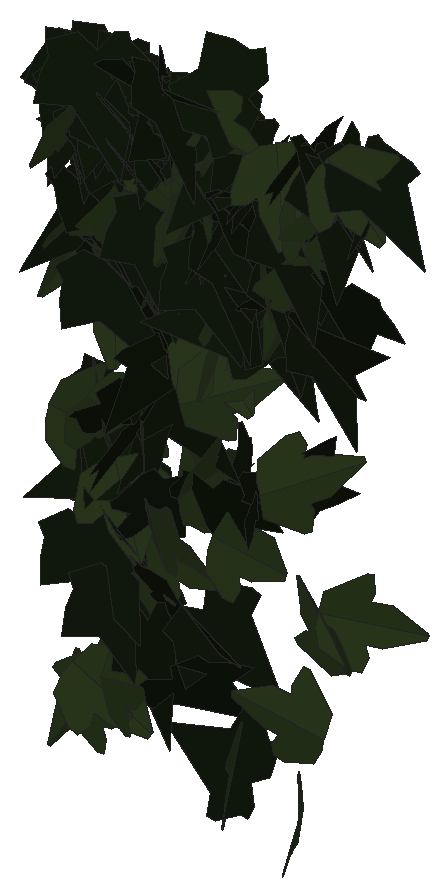
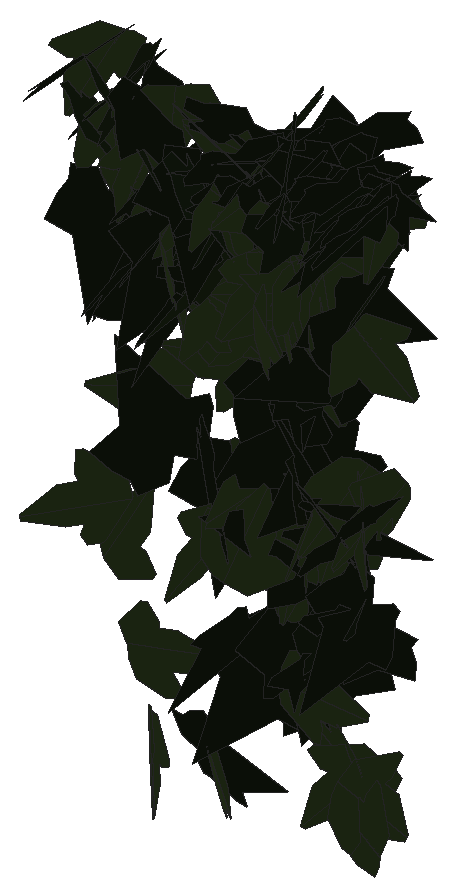
# SketchUp Ruby script. Lengths in inches.
U = 1.inch
M = Sketchup.active_model
def pt(a) = Geom::Point3d.new(a.map { |v| v * U })
def face(e, loops, mat)
  f = e.add_face(loops[0].map { |a| pt(a) })
  loops[1..].each { |l| e.add_face(l.map { |a| pt(a) }).erase! }
  f.material = f.back_material = mat if mat
  f
end
# faces: each face lists its corners as indices into pts; further lists are holes
def faces(e, pts, list, mat = nil) = list.each { |f| face(e, (f[0].is_a?(Array) ? f : [f]).map { |l| l.map { |i| pts[i] } }, mat) }
# xy, xz, yz: faces in a plane at the given z, y or x. An outline is a flat list of corners, or four numbers for a rectangle; further outlines are holes
def ring(l) = l.size == 4 ? [[l[0], l[1]], [l[2], l[1]], [l[2], l[3]], [l[0], l[3]]] : l.each_slice(2).to_a
def flat(e, list, mat, &to3) = list.each { |f| face(e, (f[0].is_a?(Array) ? f : [f]).map { |l| ring(l).map { |u, v| to3.(u, v) } }, mat) }
def xy(e, z, list, mat = nil) = flat(e, list, mat) { |x, y| [x, y, z] }
def xz(e, y, list, mat = nil) = flat(e, list, mat) { |x, z| [x, y, z] }
def yz(e, x, list, mat = nil) = flat(e, list, mat) { |y, z| [x, y, z] }
def lines(e, pts, list) = list.each { |a, b| e.add_line(pt(pts[a]), pt(pts[b])) }
# prism: a flat outline (further loops are holes) pulled along v
def prism(e, loops, v, mat = nil)
  f = face(e, loops, mat); d = Geom::Vector3d.new(v.map { |x| x * U })
  f.pushpull(f.normal.samedirection?(d) ? d.length : -d.length)
end
def box(e, o, s, mat = nil) = prism(e, [[o, [o[0] + s[0], o[1], o[2]], [o[0] + s[0], o[1] + s[1], o[2]], [o[0], o[1] + s[1], o[2]]]], [0, 0, s[2]], mat)
def at(x, y, z, deg = 0) = Geom::Transformation.translation(pt([x, y, z])) * Geom::Transformation.rotation(ORIGIN, Z_AXIS, deg.degrees)
def axes(o, x, y, z) = Geom::Transformation.new([*x, 0, *y, 0, *z, 0, *pt(o).to_a, 1])
def part(name) = M.definitions.add(name)
# library, detail: a bought-in or finely detailed component or shape, given as its bounding box
def library(name, o, s) = part(name).tap { |d| box(d.entities, o, s) }
def detail(e, o, s) = box(e.add_group.entities, o, s)
def put(e, d, t, mat = nil) = e.add_instance(d, t).tap { |i| i.material = mat if mat }
def group(e, t, mat = nil) = e.add_group.tap { |g| g.transformation = t; g.material = mat if mat }.entities
root = M.entities
M.materials.add("efeu1").color = [18, 25, 13]
M.materials.add("efeu2").color = [43, 57, 29]
c1 = part("ivyleaf_9")
p = [[1.54,2.16,1.25],[1.36,2.04,1.19],[-0.21,0.99,0.68],[-0.71,1.11,0.82],[-0.85,0.86,0.67],[-0.8,0.17,0.21],
  [-0.9,-0.01,0.1],[-0.67,-0.16,-0.02],[-0.08,-0.08,-0.05],[-0.03,-0.6,-0.4],[0.65,-0.88,-0.66],[0.83,-0.6,-0.49],
  [1.29,-0.42,-0.43],[1.8125,-0.07,-0.26],[1.21,0.44,0.15]]
faces(c1.entities,p,[[0,1,2,3,4,5,6,7,8,9,10,11,12,13,14]],"efeu1")
c2 = part("ivyleaf_10")
p = [[0,0.5,-0.03],[-0.0625,2.02,-0.43],[-0.19,2.01,-0.46],[-0.54,1.05,-0.29],[-0.52,0.625,-0.18],[-0.83,0.76,-0.28],
  [-1.16,0.64,-0.33],[-1.15,0.33,-0.24],[-0.77,-0.39,0.02],[-0.3,-0.51,0.16],[0.04,-0.48,0.23],[-0.02,2.01,-0.4375],
  [-0.06,2.01,-0.43],[0.04,-0.49,0.23],[0.67,-0.49,0.14],[1.38,0.36,-0.2],[1.375,0.51,-0.24],[0.81,0.65,-0.19],
  [0.62,0.59,-0.15],[0.6,1.09,-0.28],[0.5,1.23,-0.31]]
faces(c2.entities,p,[[0,1,2,3,4,5,6,7,8,9,10],[11,12,0,13,14,15,16,17,18,19,20]],"efeu2")
put(root,c1,axes([32.18,224.08,221.5],[-0.27203,-0.26272,-0.32707],[0.25928,0.20117,-0.37723],[0.32981,-0.37484,0.02679]))
put(root,c1,axes([31.23,224.08,223.3],[-0.1152,-0.42739,-0.23253],[0.09502,0.21459,-0.4415],[0.47718,-0.14591,0.03178]))
put(root,c2,axes([32.17,224.0625,221.27],[-0.13038,-0.10357,-0.47146],[0.46703,-0.15049,-0.09609],[-0.12199,-0.46543,0.13598]))
put(root,c1,axes([31.83,223.98,218.64],[-0.22433,0.40804,-0.18215],[0.08698,-0.16005,-0.46564],[-0.4383,-0.2406,0.00082]))
put(root,c2,axes([32.61,224.22,221.93],[-0.07898,-0.42414,0.25273],[-0.03752,-0.25004,-0.43136],[0.49229,-0.0871,0.00767]))
put(root,c1,axes([31.49,223.98,220.65],[-0.08996,-0.29949,-0.39014],[0.20065,0.33976,-0.30708],[0.44905,-0.21182,0.05905]))
put(root,c1,axes([32.98,224.03,221.29],[-0.02797,-0.42127,-0.26785],[0.00609,0.26797,-0.42209],[0.49918,-0.02688,-0.00986]))
put(root,c1,axes([34.625,224.29,222.62],[0.02741,-0.48585,0.11487],[0.03219,-0.11309,-0.48598],[0.49821,0.03404,0.02508]))
put(root,c1,axes([32.35,224.15,219.79],[-0.0278,0.28923,-0.4069],[-0.03031,-0.40776,-0.28777],[-0.49831,0.00867,0.04021]))
put(root,c2,axes([34.07,224.27,221.27],[-0.01988,-0.42647,0.26025],[0.0515,-0.26082,-0.42347],[0.49694,0.00997,0.05429]))
put(root,c2,axes([34.78,224,216.64],[-0.40489,0.1815,-0.23048],[-0.21432,0.08523,0.44362],[0.20032,0.45803,0.00878]))
put(root,c2,axes([33,223.79,219.55],[0.07126,0.05888,-0.49138],[0.42437,0.24814,0.09128],[0.25461,-0.43007,-0.01461]))
put(root,c2,axes([34.31,224.1,215.46],[0.09993,0.06613,0.48543],[-0.45931,-0.15971,0.11631],[0.17044,-0.46917,0.02883]))
put(root,c1,axes([31.92,224.15,215.96],[-0.24572,-0.07659,-0.42867],[0.41218,0.11787,-0.25733],[0.14047,-0.47983,0.00521]))
put(root,c2,axes([32.2,223.96,217.55],[-0.45407,0.20337,0.0496],[-0.04555,0.01965,-0.49753],[-0.20432,-0.45635,0.00068]))
put(root,c1,axes([32.66,223.76,215.68],[0.37035,0.32086,0.09943],[0.0771,0.06286,-0.49],[-0.32695,0.37828,-0.00292]))
put(root,c1,axes([33.56,224.31,220.49],[-0.31118,-0.02444,0.3906],[-0.36704,-0.15496,-0.3021],[0.13582,-0.47475,0.0785]))
put(root,c1,axes([31.64,224.02,222.13],[0.45095,-0.21582,0.00813],[0.01029,0.00268,-0.49989],[0.21573,0.45101,0.00686]))
put(root,c2,axes([34.18,223.77,218.77],[0.0849,0.02416,-0.49215],[0.37014,0.32652,0.07988],[0.32525,-0.37789,0.03756]))
put(root,c2,axes([32.67,224.32,221.98],[-0.06079,-0.39812,0.29632],[-0.00785,-0.29772,-0.40162],[0.49623,-0.05348,0.02995]))
put(root,c2,axes([30.93,223.93,222.47],[-0.06934,-0.43109,-0.24362],[0.0283,0.24215,-0.43654],[0.49436,-0.07432,-0.00918]))
put(root,c2,axes([32.93,223.9375,220.16],[0.301,0.28662,0.27794],[0.20478,0.18797,-0.41561],[-0.34273,0.36403,-0.00423]))
put(root,c1,axes([32.96,224.28,221.27],[0.15913,-0.46617,0.08584],[0.03221,-0.0797,-0.49255],[0.47291,0.16229,0.00467]))
put(root,c2,axes([32.12,224.12,217.07],[0.0067,-0.02964,0.49908],[0.49965,0.01781,-0.00565],[-0.01744,0.4988,0.02985]))
put(root,c2,axes([31.26,224.24,215.03],[0.11189,-0.07572,-0.4814],[0.39978,-0.26819,0.13511],[-0.27867,-0.41514,0.00053]))
put(root,c1,axes([33.16,223.98,221.75],[-0.29035,0.40675,0.01591],[-0.00936,0.01286,-0.49975],[-0.40695,-0.2905,0.00015]))
put(root,c2,axes([31.57,224.03,217.82],[0.37927,0.2919,0.14475],[0.11477,0.0882,-0.47859],[-0.30494,0.39625,-0.0001]))
put(root,c1,axes([31.69,224.35,218.07],[-0.41121,-0.10849,0.26293],[-0.24916,-0.08554,-0.42497],[0.1372,-0.48053,0.01629]))
put(root,c2,axes([33.16,224.27,220.39],[0.08514,0.40327,-0.28306],[-0.14399,-0.25435,-0.40568],[-0.47119,0.15059,0.07282]))
put(root,c1,axes([31.86,223.95,220.48],[0.34064,0.02716,-0.36501],[-0.36578,0.00748,-0.3408],[-0.01305,0.49921,0.02497]))
put(root,c1,axes([32,224.2,216.39],[0.33736,-0.20812,0.30474],[0.24943,-0.1757,-0.39612],[0.27197,0.4193,-0.01472]))
put(root,c1,axes([31.93,224.22,222.58],[-0.35338,0.06575,0.34757],[-0.34331,0.0546,-0.35938],[-0.08521,-0.49264,0.00655]))
put(root,c2,axes([33.86,224.11,222.75],[0.32841,0.37527,0.03633],[0.02078,0.03009,-0.49866],[-0.37645,0.32904,0.00417]))
put(root,c2,axes([34.91,223.95,223.04],[0.19002,0.39023,0.24822],[0.09231,0.23095,-0.43375],[-0.45318,0.21067,0.01573]))
put(root,c1,axes([30.84,224.13,221.52],[0.32306,-0.35606,-0.13731],[-0.07801,0.1145,-0.48042],[0.37356,0.33183,0.01843]))
put(root,c1,axes([32.03,224.36,223.03],[0.16678,-0.46107,0.09798],[0.04932,-0.0863,-0.49002],[0.46878,0.17312,0.01669]))
put(root,c1,axes([31.42,224.41,222.34],[0.1051,-0.32874,0.36178],[0.23849,-0.28853,-0.33147],[0.4267,0.24224,0.09616]))
put(root,c1,axes([33.83,224.4,221.11],[0.10544,-0.47871,0.09857],[0.01472,-0.09768,-0.49014],[0.48853,0.10626,-0.00651]))
put(root,c2,axes([34.26,223.99,214.37],[0.17023,-0.33902,-0.32571],[-0.11336,0.30659,-0.37836],[0.45626,0.20267,0.02752]))
put(root,c1,axes([33.02,224.02,218.19],[0.3815,0.2155,-0.24087],[-0.20443,-0.12773,-0.43806],[-0.25033,0.43272,-0.00935]))
put(root,c2,axes([30.98,224.46,214.89],[-0.04317,-0.35537,0.34907],[-0.01288,-0.34946,-0.35736],[0.49797,-0.03985,0.02102]))
put(root,c1,axes([31.27,224.45,216.9],[0.41424,-0.19556,-0.2004],[0.18295,-0.08187,0.45807],[-0.21198,-0.45283,0.00373]))
put(root,c2,axes([31.46,224.28,221.3125],[-0.09706,-0.48688,0.05938],[-0.00407,-0.05973,-0.4964],[0.49047,-0.09685,0.00764]))
put(root,c1,axes([34.21,224.22,220.4],[0.39013,0.09559,-0.29777],[0.27461,0.12309,0.3993],[0.14964,-0.47509,0.04354]))
put(root,c2,axes([31.41,224.2,220.3],[0.34404,0.36273,-0.00798],[-0.01058,-0.00097,-0.49989],[-0.36267,0.34413,0.00701]))
put(root,c1,axes([31.18,224.4,220.31],[0.17008,-0.29493,0.36618],[0.29053,-0.24024,-0.32845],[0.36968,0.3245,0.08965]))
put(root,c1,axes([31.46,224.25,216.3],[-0.11886,-0.39196,-0.28678],[0.08341,0.27438,-0.40958],[0.47845,-0.14521,0.00016]))
put(root,c1,axes([33.87,224.38,221.86],[0.09409,-0.48992,-0.03358],[0.00509,0.03516,-0.49874],[0.49104,0.09351,0.0116]))
put(root,c1,axes([31.02,224.23,216.91],[-0.15241,-0.26772,-0.39382],[0.25658,0.30218,-0.30472],[0.40117,-0.29498,0.04527]))
put(root,c1,axes([31.6,224.48,220.4],[0.09669,-0.21546,0.44071],[0.23174,-0.37585,-0.23459],[0.43238,0.24963,0.02718]))
put(root,c1,axes([31.51,223.87,218.89],[0.32121,0.32666,0.20028],[0.13184,0.15117,-0.458],[-0.35978,0.34704,0.01098]))
put(root,c1,axes([30.83,224.4375,222.87],[-0.41646,-0.20356,-0.18742],[0.18892,0.03826,-0.46135],[0.20217,-0.45508,0.04504]))
put(root,c2,axes([34.61,224.3,222.29],[-0.19346,-0.4585,0.04851],[-0.01771,-0.04518,-0.49764],[0.46072,-0.19426,0.00124]))
put(root,c1,axes([31.92,223.93,217.57],[0.16242,0.37354,-0.28997],[0.03476,0.29634,0.40121],[0.47161,-0.15049,0.0703]))
put(root,c2,axes([30.9,223.92,218.53],[-0.01665,0.30465,0.39612],[-0.01395,0.3959,-0.30507],[-0.49953,-0.02121,-0.00468]))
put(root,c1,axes([33.8,224.25,218.28],[0.41157,0.28149,0.03704],[-0.04419,-0.00091,0.49804],[0.28046,-0.41323,0.02413]))
put(root,c1,axes([33.03,224.3,221.7],[0.37412,-0.33171,-0.00134],[-0.00102,0.00086,-0.5],[0.33171,0.37412,-0.00003]))
put(root,c1,axes([33.39,224.15,214.45],[-0.19958,0.15027,0.43311],[-0.34705,0.25912,-0.24983],[-0.29954,-0.40035,0.00087]))
put(root,c2,axes([34.88,224.01,217.14],[0.05888,0.0587,0.49304],[0.31152,0.38225,-0.08272],[-0.38664,0.31692,0.00844]))
put(root,c2,axes([32.02,224.34,220.74],[0.20833,-0.45428,-0.01524],[-0.00584,0.01409,-0.49977],[0.4545,0.20841,0.00057]))
put(root,c1,axes([31.85,224.68,222.53],[-0.07311,-0.27036,0.4142],[-0.01404,-0.41739,-0.27493],[0.49443,-0.05183,0.05344]))
put(root,c2,axes([30.89,224.375,220.79],[0.11653,0.41771,-0.24888],[-0.27037,-0.15705,-0.39018],[-0.40413,0.22551,0.18927]))
put(root,c2,axes([33.73,224.17,221.31],[-0.1892,0.45984,0.05246],[-0.02418,0.04678,-0.49722],[-0.46219,-0.19068,0.00454]))
put(root,c2,axes([32.98,224.47,214.66],[0.26883,-0.36443,0.21196],[0.1538,-0.14929,-0.45173],[0.39253,0.30807,0.03183]))
put(root,c1,axes([34.26,224.37,222.89],[0.32172,-0.38266,0.00816],[0.00196,-0.009,-0.49992],[0.38274,0.3217,-0.00429]))
put(root,c1,axes([31.05,224.63,221.24],[-0.00777,-0.01405,-0.49974],[0.08149,-0.49315,0.0126],[-0.49325,-0.08125,0.00996]))
put(root,c2,axes([31.23,224.11,218.68],[-0.21503,-0.31132,-0.32686],[0.22208,0.24224,-0.37682],[0.39299,-0.30724,0.0341]))
put(root,c2,axes([32.73,224.08,221.77],[0.03742,0.00529,-0.49857],[-0.36997,0.33547,-0.0242],[0.33425,0.37072,0.02902]))
put(root,c1,axes([34.28,224.42,220.59],[0.16986,-0.46602,-0.06306],[-0.01739,0.06078,-0.49599],[0.46994,0.17069,0.00444]))
put(root,c1,axes([34.93,224.37,223.08],[0.18263,-0.4489,-0.12302],[0.08248,0.16128,-0.46603],[0.45808,0.14993,0.13296]))
put(root,c2,axes([31.08,224.1,215],[0.21037,0.27797,0.35843],[0.20903,0.29124,-0.34855],[-0.40255,0.2965,0.00633]))
put(root,c1,axes([31.72,224.44,218.49],[-0.47134,0.07294,-0.15005],[0.14836,-0.0225,-0.47695],[-0.07633,-0.49414,-0.00043]))
put(root,c1,axes([32.22,224.49,222.13],[-0.30491,-0.09532,-0.38463],[0.3884,0.02433,-0.31393],[0.07856,-0.49023,0.05921]))
put(root,c1,axes([32.94,224.6875,222.42],[-0.37886,-0.3068,0.11109],[0.02379,-0.19574,-0.45948],[0.32543,-0.34287,0.16291]))
put(root,c1,axes([31.32,224.31,222.74],[0.24389,-0.13548,0.41493],[0.41199,-0.08554,-0.27009],[0.14417,0.47363,0.06991]))
put(root,c1,axes([31.7,224.66,222.625],[-0.01673,-0.46819,0.17471],[-0.00392,-0.17468,-0.46848],[0.4997,-0.01705,0.00217]))
put(root,c1,axes([34.08,224.4,222.9],[-0.20709,0.36849,-0.26708],[0.13618,-0.22981,-0.42266],[-0.43425,-0.2478,-0.00518]))
put(root,c1,axes([32.75,224.2,216.4],[0.15837,-0.29336,-0.37264],[-0.0676,0.37489,-0.32386],[0.46941,0.15296,0.07908]))
put(root,c1,axes([34.99,224.31,222.4],[-0.3661,0.34016,0.01618],[-0.01293,0.00985,-0.49974],[-0.3403,-0.36632,0.00158]))
put(root,c2,axes([31.32,224.49,221.25],[0.03536,-0.48992,0.09343],[0.10655,-0.08408,-0.48123],[0.48723,0.05394,0.09845]))
put(root,c1,axes([31.95,224.31,219.08],[-0.06977,-0.03887,-0.49358],[0.3874,0.30611,-0.07887],[0.30831,-0.39343,-0.01259]))
put(root,c2,axes([32.59,224.47,222.66],[-0.05282,-0.03222,-0.49616],[0.45614,-0.2017,-0.03546],[-0.19786,-0.45638,0.0507]))
put(root,c1,axes([33.38,224.2,218.46],[0.04569,-0.0129,-0.49774],[-0.49518,0.05111,-0.04678],[0.05208,0.49721,-0.0081]))
put(root,c2,axes([31.97,224.43,221.92],[0.49845,0.03906,0.00491],[0.00447,0.00577,-0.49995],[-0.03912,0.49844,0.0054]))
put(root,c2,axes([31.86,224.34,215.93],[0.03564,-0.0176,-0.49842],[-0.48047,0.13276,-0.03904],[0.13371,0.48173,-0.00745]))
put(root,c1,axes([33.13,224.58,222.84],[-0.47412,0.00609,-0.15866],[0.15517,-0.08809,-0.46708],[-0.03364,-0.49214,0.08164]))
put(root,c2,axes([32.54,224.02,222.05],[-0.00833,-0.06616,-0.49553],[0.12036,0.48076,-0.06621],[0.48523,-0.12039,0.00791]))
put(root,c1,axes([31.11,224.65,222.9],[-0.30822,-0.38853,-0.06362],[0.0783,0.0187,-0.49348],[0.38584,-0.31416,0.04932]))
put(root,c2,axes([31.18,224.2,218.48],[-0.24143,0.16808,0.4043],[-0.36297,0.18138,-0.29216],[-0.24488,-0.43457,0.03443]))
put(root,c2,axes([30.7,224.49,214.4],[-0.15771,0.02127,0.474],[0.47228,-0.04092,0.15898],[0.04555,0.49787,-0.00718]))
put(root,c2,axes([32.13,224.64,220.74],[0.17628,-0.39926,0.24396],[0.1309,-0.20821,-0.43533],[0.44921,0.21735,0.03112]))
put(root,c2,axes([32.71,224.05,218.08],[0.10533,-0.02236,0.48827],[-0.13973,0.47726,0.052],[-0.46838,-0.1474,0.09429]))
put(root,c1,axes([31.96,224.39,219.46],[0.23868,-0.14902,0.41331],[-0.26747,0.32386,0.27124],[-0.34855,-0.35058,0.07488]))
put(root,c1,axes([30.59,224.67,222.78],[-0.03404,-0.49877,-0.00827],[-0.00198,0.00842,-0.49993],[0.49884,-0.034,-0.00255]))
put(root,c2,axes([31.55,224.6,218.34],[-0.12596,0.36636,-0.31609],[0.10349,-0.29867,-0.38741],[-0.47268,-0.16302,-0.0006]))
put(root,c1,axes([34.7,224.3,221.29],[0.38261,0.15461,-0.28232],[-0.26361,-0.10117,-0.41265],[-0.18472,0.46461,0.00409]))
put(root,c1,axes([30.96,224.78,218.38],[-0.09262,-0.47275,0.13391],[-0.0169,-0.13312,-0.48166],[0.49106,-0.09375,0.00867]))
put(root,c2,axes([31.67,224.57,221.32],[-0.07064,-0.48863,0.07904],[-0.0228,-0.07654,-0.49358],[0.49446,-0.07333,-0.01147]))
put(root,c1,axes([32.38,224.58,222.3125],[-0.21825,-0.37633,-0.24646],[0.13411,0.20705,-0.43491],[0.4294,-0.25595,0.01056]))
put(root,c1,axes([30.71,224.74,222.46],[-0.05477,-0.49378,0.0564],[0.00532,-0.05732,-0.49667],[0.49696,-0.05381,0.01153]))
put(root,c1,axes([30.68,224.46,222.7],[0.11932,-0.41388,-0.25391],[0.01902,0.26524,-0.42342],[0.48518,0.09139,0.07904]))
put(root,c2,axes([34.1,224.3,222.2],[0.01386,0.47274,0.16225],[-0.01448,0.16262,-0.47259],[-0.4996,0.00841,0.0182]))
put(root,c1,axes([33.21,224.28,222.04],[0.25082,0.41312,-0.12815],[-0.06476,-0.1106,-0.48329],[-0.42766,0.25904,-0.00197]))
put(root,c1,axes([32.69,224.74,222.11],[-0.1767,-0.46766,0.00829],[-0.0054,-0.00683,-0.49992],[0.4677,-0.17676,-0.00263]))
put(root,c1,axes([30.97,224.72,222.95],[-0.14301,-0.47795,-0.03339],[0.0133,0.03087,-0.49887],[0.47893,-0.14357,0.00388]))
put(root,c2,axes([31.8,224.41,221.64],[0.30253,-0.27964,-0.28333],[-0.20274,0.19802,-0.41193],[0.34259,0.36413,0.00643]))
put(root,c1,axes([34.64,224.28,222.62],[-0.25664,0.34308,0.25774],[-0.14494,0.21336,-0.42833],[-0.40389,-0.29457,-0.01006]))
put(root,c2,axes([33.12,224.16,217.44],[0.0354,0.30225,0.39673],[0.00029,0.39771,-0.30303],[-0.49874,0.02168,0.02799]))
put(root,c2,axes([33.6,224.53,221.01],[0.22442,-0.44358,-0.0536],[-0.02194,0.04897,-0.49711],[0.44627,0.22548,0.00252]))
put(root,c1,axes([31.1,224.24,220.43],[0.40382,0.10435,0.27575],[0.2598,0.09515,-0.41647],[-0.13939,0.47964,0.02263]))
put(root,c2,axes([32.74,224.72,222.1875],[0.06533,0.35294,-0.34809],[-0.10272,-0.33384,-0.35777],[-0.48495,0.11826,0.02889]))
put(root,c1,axes([31.7,224.77,222.84],[0.06862,-0.03092,-0.4943],[0.46383,-0.17094,0.07508],[-0.17364,-0.46885,0.00522]))
put(root,c2,axes([31.91,224.46,221.08],[-0.13924,-0.03287,-0.47909],[0.4802,-0.00504,-0.13922],[0.00432,-0.49889,0.03297]))
put(root,c2,axes([32.125,224.4,221.16],[-0.3879,-0.1221,-0.2909],[0.2768,0.08949,-0.40666],[0.15138,-0.47653,-0.00183]))
put(root,c1,axes([31.07,224.42,222.18],[0.24597,-0.34782,-0.26177],[-0.02573,0.28852,-0.40755],[0.43456,0.21396,0.12403]))
put(root,c1,axes([30.85,224.36,217.3125],[0.48282,0.0717,-0.10836],[-0.10811,-0.00961,-0.48808],[-0.07207,0.49474,0.00623]))
put(root,c1,axes([31.625,224.65,222.21],[0.31478,-0.29918,0.24781],[0.20738,-0.14029,-0.4328],[0.32849,0.37525,0.03577]))
put(root,c1,axes([33.31,224.51,222.18],[-0.3402,0.36005,-0.06802],[0.03498,-0.06048,-0.49509],[-0.36475,-0.34162,0.01597]))
put(root,c1,axes([32.89,224.69,223.06],[-0.40483,0.05125,0.28894],[-0.29307,-0.04554,-0.40254],[-0.01494,-0.49528,0.06691]))
put(root,c1,axes([32.4375,224.75,222.81],[-0.204,-0.44305,-0.10993],[0.03957,0.1028,-0.48772],[0.45477,-0.20769,-0.00688]))
put(root,c1,axes([33.42,224.55,220.52],[0.20274,-0.39797,-0.22476],[-0.11263,0.19479,-0.44651],[0.44296,0.23168,-0.01066]))
put(root,c1,axes([32.93,224.37,221.1],[0.41222,-0.17128,-0.22525],[-0.12393,0.24852,-0.41579],[0.25439,0.39862,0.16243]))
put(root,c2,axes([32.56,224.66,217.45],[-0.46198,-0.07401,-0.17633],[-0.17444,-0.02585,0.46787],[-0.07837,0.49382,-0.00194]))
put(root,c1,axes([30.8,224.77,222.61],[0.07425,-0.49431,-0.01218],[0.00174,0.01257,-0.49984],[0.49445,0.07419,0.00358]))
put(root,c1,axes([30.92,224.39,222.8],[0.46959,0.07816,-0.1529],[-0.1582,0.02383,-0.47371],[-0.06676,0.49328,0.04712]))
put(root,c1,axes([33.67,224.23,220.96],[0.2067,0.42147,0.17215],[0.07741,0.15377,-0.46943],[-0.44865,0.22071,-0.00168]))
